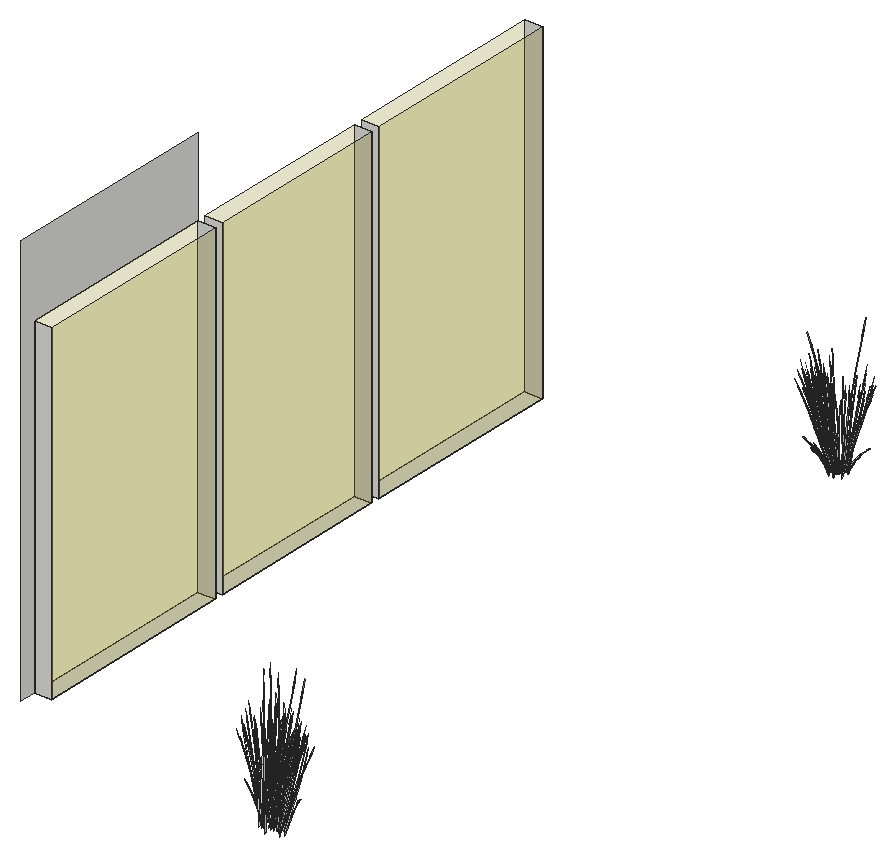
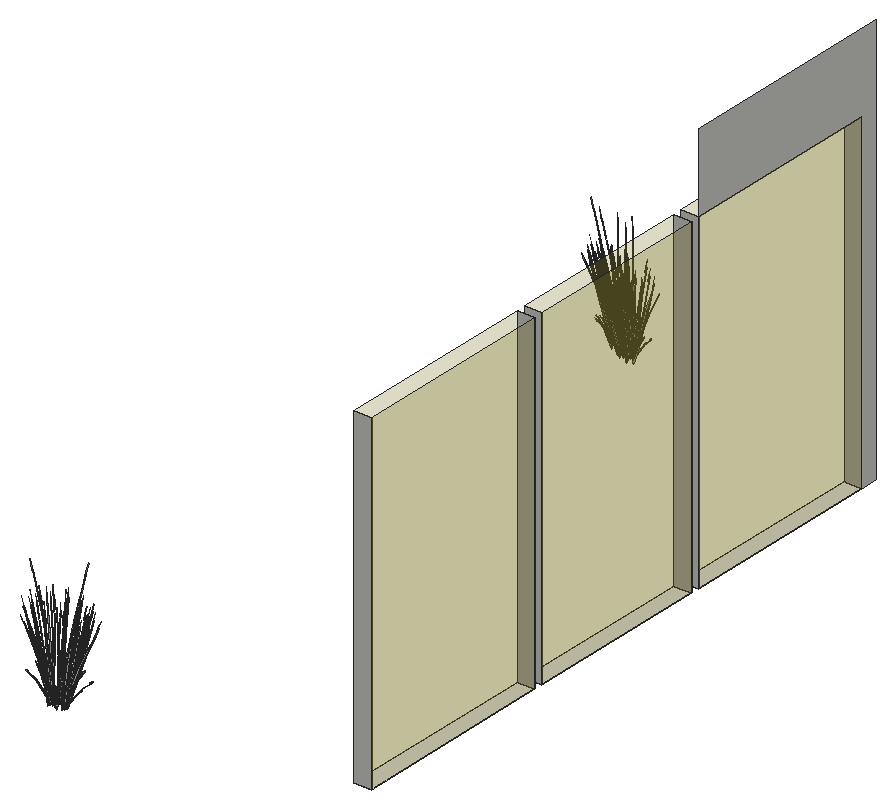
# SketchUp Ruby script. Lengths in inches.
U = 1.inch
M = Sketchup.active_model
def pt(a) = Geom::Point3d.new(a.map { |v| v * U })
def face(e, loops, mat)
  f = e.add_face(loops[0].map { |a| pt(a) })
  loops[1..].each { |l| e.add_face(l.map { |a| pt(a) }).erase! }
  f.material = f.back_material = mat if mat
  f
end
# faces: each face lists its corners as indices into pts; further lists are holes
def faces(e, pts, list, mat = nil) = list.each { |f| face(e, (f[0].is_a?(Array) ? f : [f]).map { |l| l.map { |i| pts[i] } }, mat) }
# xy, xz, yz: faces in a plane at the given z, y or x. An outline is a flat list of corners, or four numbers for a rectangle; further outlines are holes
def ring(l) = l.size == 4 ? [[l[0], l[1]], [l[2], l[1]], [l[2], l[3]], [l[0], l[3]]] : l.each_slice(2).to_a
def flat(e, list, mat, &to3) = list.each { |f| face(e, (f[0].is_a?(Array) ? f : [f]).map { |l| ring(l).map { |u, v| to3.(u, v) } }, mat) }
def xy(e, z, list, mat = nil) = flat(e, list, mat) { |x, y| [x, y, z] }
def xz(e, y, list, mat = nil) = flat(e, list, mat) { |x, z| [x, y, z] }
def yz(e, x, list, mat = nil) = flat(e, list, mat) { |y, z| [x, y, z] }
def lines(e, pts, list) = list.each { |a, b| e.add_line(pt(pts[a]), pt(pts[b])) }
# prism: a flat outline (further loops are holes) pulled along v
def prism(e, loops, v, mat = nil)
  f = face(e, loops, mat); d = Geom::Vector3d.new(v.map { |x| x * U })
  f.pushpull(f.normal.samedirection?(d) ? d.length : -d.length)
end
def box(e, o, s, mat = nil) = prism(e, [[o, [o[0] + s[0], o[1], o[2]], [o[0] + s[0], o[1] + s[1], o[2]], [o[0], o[1] + s[1], o[2]]]], [0, 0, s[2]], mat)
def at(x, y, z, deg = 0) = Geom::Transformation.translation(pt([x, y, z])) * Geom::Transformation.rotation(ORIGIN, Z_AXIS, deg.degrees)
def axes(o, x, y, z) = Geom::Transformation.new([*x, 0, *y, 0, *z, 0, *pt(o).to_a, 1])
def part(name) = M.definitions.add(name)
# library, detail: a bought-in or finely detailed component or shape, given as its bounding box
def library(name, o, s) = part(name).tap { |d| box(d.entities, o, s) }
def detail(e, o, s) = box(e.add_group.entities, o, s)
def put(e, d, t, mat = nil) = e.add_instance(d, t).tap { |i| i.material = mat if mat }
def group(e, t, mat = nil) = e.add_group.tap { |g| g.transformation = t; g.material = mat if mat }.entities
root = M.entities
M.materials.add("Glass_Basic_01").color = [186, 175, 42]
M.materials["Glass_Basic_01"].alpha = 0.25
M.materials.add("LightPink_Translucent").color = [144, 107, 117]
M.materials["LightPink_Translucent"].alpha = 0.75
c1 = part("blade")
p = [[2.15,0.21,22],[0,0.17,0],[0.09,0.45,0],[2.18,0.31,22],[2.29,0.31,22],[0.38,0.45,0],
  [2.48,0.24,33],[2.49,0.24,33],[2.48,0.22,33]]
faces(c1.entities,p,[[0,1,2,3],[4,5,2,3],[6,3,4,7],[8,0,3,6]])
c2 = part("seeds")
p = [[0.3,-0.1,1.38],[-0.01,-0.03,1.59],[-0.01,-0.03,0.03],[0.14,-0.07,-0.07],[0.29,-0.03,3],[0.15,0.01,3.11]]
faces(c2.entities,p,[[0,1,2,3],[1,0,4,5]],"LightPink_Translucent")
c3 = part("blade with seeds")
put(c3.entities,c1,at(0,0,0))
put(c3.entities,c2,axes([2.4,0.25,30.99],[1.5799,-0.05474,1.17369],[-0.12525,1.92788,0.29478],[-0.07173,-0.02425,1.56792]))
xy(root,51,[[241,49,247,119],[241,122,247,186],[241,189,247,259]])
xz(root,49,[[241,51,247,165]])
xz(root,119,[[241,51,247,165]])
xz(root,122,[[241,51,247,165]])
xz(root,186,[[241,51,247,165]])
xz(root,189,[[241,51,247,165]])
xz(root,259,[[241,51,247,165]])
yz(root,241,[[43,51,43,192,119,192,119,165,49,165,49,51]])
yz(root,241,[[49,51,119,165],[122,51,186,165],[189,51,259,165]],"Glass_Basic_01")
yz(root,247,[[49,51,119,165],[122,51,186,165],[189,51,259,165]],"Glass_Basic_01")
put(root,c3,axes([336.58,28.07,50.51],[-0.01379,-0.36791,1.24828],[0.62424,0.09537,0.52853],[-0.14764,0.20132,1.17828]))
put(root,c3,axes([336.63,29.49,52.14],[0.49824,-0.09289,-0.45151],[0.08716,0.35177,-0.34973],[0.13382,0.10081,0.86392]))
put(root,c3,axes([336.7,30.62,50.44],[0.21042,-0.1771,1.01491],[0.08303,0.28036,0.74569],[-0.15207,0.0502,0.22354]))
put(root,c3,axes([341.77,30.29,52],[0.28729,0.24465,-0.31292],[-0.32804,0.23159,0.40398],[0.16667,0.03524,0.77298]))
put(root,c3,axes([336.83,32.29,52.4],[0.44368,-0.17257,-0.62776],[0.24726,0.35524,0.07576],[0.21437,-0.04035,0.88802]))
put(root,c3,axes([337.49,29.85,52],[-0.43951,0.05584,-0.31292],[-0.11606,-0.31924,0.40398],[-0.12595,0.08575,0.77298]))
put(root,c3,axes([334,28.74,51.43],[0.09401,-0.13431,1.51428],[0.3944,0.27795,0.12244],[-0.17792,0.17323,0.64734]))
put(root,c3,axes([340.73,29.67,51.43],[-0.18755,-0.06732,1.51428],[0.38813,-0.28243,0.12244],[0.24191,0.12741,0.64734]))
put(root,c3,axes([340.77,28.78,51.95],[-0.4363,-0.20303,1.22187],[0.46069,-0.31611,0.5272],[0.14077,0.1905,1.18105]))
put(root,c3,axes([334.11,29.5,52],[-0.34164,0.20573,-0.31292],[-0.3234,-0.23491,0.40398],[-0.04921,0.11936,0.77298]))
put(root,c3,axes([335.1,29.67,52.45],[0.49409,-0.18193,-0.10745],[0.24281,0.32289,-0.59638],[0.06519,0.13607,0.90619]))
put(root,c3,axes([337.625,29.64,52.45],[0.46706,0.21546,-0.10745],[-0.26908,0.31203,-0.59638],[-0.13196,0.10846,0.90619]))
put(root,c3,axes([341.43,30.43,50.44],[-0.28429,-0.11236,1.01491],[0.36709,-0.11416,0.74569],[0.09901,0.0967,0.22354]))
put(root,c3,axes([334.33,30.3,50.44],[-0.01307,-0.23234,1.01491],[0.32652,0.16572,0.74569],[-0.06422,0.11074,0.22354]))
put(root,c3,axes([337.21,32.32,52],[0.41962,0.10901,-0.31292],[-0.12239,0.31802,0.40398],[0.16894,-0.02916,0.77298]))
put(root,c3,axes([340.43,30.75,52.45],[0.30087,-0.33447,-0.10745],[0.43572,0.19269,-0.59638],[0.15146,0.0945,0.90619]))
put(root,c3,axes([338.25,29.54,51.43],[0.12611,-0.12006,1.51428],[0.31843,0.32408,0.12244],[-0.2184,0.14759,0.64734]))
put(root,c3,axes([332.27,31.82,52],[-0.41962,-0.10901,-0.31292],[0.12239,-0.31802,0.40398],[-0.16894,0.02916,0.77298]))
put(root,c3,axes([337.86,29.89,52.14],[0.12971,0.3568,-0.45151],[-0.49122,0.06241,-0.34973],[-0.14077,0.09583,0.86392]))
put(root,c3,axes([334.45,29.4,52.42],[0.36145,0.26255,-0.50118],[-0.38183,0.22994,-0.3882],[-0.055,0.1334,0.95895]))
put(root,c3,axes([336.0625,31.93,51.43],[-0.20943,0.00885,1.51428],[0.13893,-0.38357,0.12244],[0.29846,0.02372,0.64734]))
put(root,c3,axes([340.74,29.17,50.51],[-0.01379,-0.36791,1.24828],[0.62424,0.09537,0.52853],[-0.14764,0.20132,1.17828]))
put(root,c3,axes([335.52,29.66,52.14],[0.49634,0.09796,-0.45151],[-0.17013,0.33585,-0.34973],[0.04551,0.13522,0.86392]))
put(root,c3,axes([335.8,28.96,51.43],[-0.11542,-0.12546,1.51428],[0.53333,-0.10562,0.12244],[0.12054,0.19696,0.64734]))
put(root,c3,axes([340.79,30.59,52.14],[0.49824,-0.09289,-0.45151],[0.08716,0.35177,-0.34973],[0.13382,0.10081,0.86392]))
put(root,c3,axes([335.3,29.86,52],[-0.15222,0.30049,-0.31292],[-0.44409,-0.08764,0.40398],[0.04072,0.12098,0.77298]))
put(root,c3,axes([334.34,29.28,52.72],[-0.01314,0.36145,-0.69681],[-0.55324,-0.02428,0.08409],[-0.05838,0.15313,0.9857]))
put(root,c3,axes([334.86,29.03,51.43],[-0.01236,-0.14998,1.51428],[0.53562,0.09949,0.12244],[-0.03313,0.21373,0.64734]))
put(root,c3,axes([333.55,31.76,50.95],[0.14352,-0.05653,1.56454],[0.04949,0.39467,0.12244],[-0.31087,0.05237,0.55918]))
put(root,c3,axes([338.1,32.39,50.44],[-0.31197,0.06451,1.01491],[0.14684,-0.26661,0.74569],[0.1655,0.01824,0.22354]))
put(root,c3,axes([338.16,29.84,51.43],[0.09401,-0.13431,1.51428],[0.3944,0.27795,0.12244],[-0.17792,0.17323,0.64734]))
put(root,c3,axes([335.34,29.59,52.4],[0.24099,0.31773,-0.62776],[-0.49607,0.17707,0.07576],[0.05635,0.15352,0.88802]))
put(root,c3,axes([338.27,30.59,52],[-0.34164,0.20573,-0.31292],[-0.3234,-0.23491,0.40398],[-0.04921,0.11936,0.77298]))
put(root,c3,axes([339.25,30.77,52.45],[0.49409,-0.18193,-0.10745],[0.24281,0.32289,-0.59638],[0.06519,0.13607,0.90619]))
put(root,c3,axes([332.01,32.03,52.17],[-0.08245,0.05073,1.54581],[0.00701,0.37067,-0.24447],[-0.18899,0.0482,0.12397]))
put(root,c3,axes([332.5625,31.98,52.14],[-0.13679,0.35544,-0.45151],[-0.46898,-0.12183,-0.34973],[-0.18882,0.03259,0.86392]))
put(root,c3,axes([332.54,31.67,52.45],[0.25405,0.35383,-0.10745],[-0.45089,0.17388,-0.59638],[-0.19001,0.04668,0.90619]))
put(root,c3,axes([337.55,33.21,51.47],[-0.09664,-0.32847,-0.03085],[0.45676,-0.07551,-0.13989],[0.09538,0.02082,0.4614]))
put(root,c3,axes([338.48,31.39,50.44],[-0.01307,-0.23234,1.01491],[0.32652,0.16572,0.74569],[-0.06422,0.11074,0.22354]))
put(root,c3,axes([336.37,33.2,52.45],[0.02704,-0.39739,-0.10745],[0.51189,0.01086,-0.59638],[0.19715,0.0276,0.90619]))
put(root,c3,axes([338.61,30.5,52.42],[0.36145,0.26255,-0.50118],[-0.38183,0.22994,-0.3882],[-0.055,0.1334,0.95895]))
put(root,c3,axes([339.68,30.75,52.14],[0.49634,0.09796,-0.45151],[-0.17013,0.33585,-0.34973],[0.04551,0.13522,0.86392]))
put(root,c3,axes([334.15,29.79,50.97],[0.01109,-0.20172,1.3638],[0.49896,0.10655,0.18846],[-0.04323,0.21498,0.64398]))
put(root,c3,axes([339.96,30.06,51.43],[-0.11542,-0.12546,1.51428],[0.53333,-0.10562,0.12244],[0.12054,0.19696,0.64734]))
put(root,c3,axes([339.45,30.96,52],[-0.15222,0.30049,-0.31292],[-0.44409,-0.08764,0.40398],[0.04072,0.12098,0.77298]))
put(root,c3,axes([336.82,32.96,52.17],[0.10831,-0.00661,1.54581],[0.29709,-0.30358,-0.24447],[0.19266,0.04007,0.12397]))
put(root,c3,axes([338.49,30.375,52.72],[-0.01314,0.36145,-0.69681],[-0.55324,-0.02428,0.08409],[-0.05838,0.15313,0.9857]))
put(root,c3,axes([332.55,32.16,51.43],[0.17519,-0.08265,1.51428],[0.14749,0.38193,0.12244],[-0.27504,0.08632,0.64734]))
put(root,c3,axes([339.02,30.12,51.43],[-0.01236,-0.14998,1.51428],[0.53562,0.09949,0.12244],[-0.03313,0.21373,0.64734]))
put(root,c3,axes([336.4,33.01,52.4],[0.50473,0.00941,-0.62776],[-0.0339,0.39618,0.07576],[0.21383,0.04181,0.88802]))
put(root,c3,axes([339.5,30.6875,52.4],[0.24099,0.31773,-0.62776],[-0.49607,0.17707,0.07576],[0.05635,0.15352,0.88802]))
put(root,c3,axes([331.63,33.5,50.44],[0.21042,-0.1771,1.01491],[0.08303,0.28036,0.74569],[-0.15207,0.0502,0.22354]))
put(root,c3,axes([336.7,33.17,52],[0.28729,0.24465,-0.31292],[-0.32804,0.23159,0.40398],[0.16667,0.03524,0.77298]))
put(root,c3,axes([332.43,32.73,52],[-0.43951,0.05584,-0.31292],[-0.11606,-0.31924,0.40398],[-0.12595,0.08575,0.77298]))
put(root,c3,axes([338.31,30.89,50.97],[0.01109,-0.20172,1.3638],[0.49896,0.10655,0.18846],[-0.04323,0.21498,0.64398]))
put(root,c3,axes([335.67,32.54,51.43],[-0.18755,-0.06732,1.51428],[0.38813,-0.28243,0.12244],[0.24191,0.12741,0.64734]))
put(root,c3,axes([335.7,31.66,51.95],[-0.4363,-0.20303,1.22187],[0.46069,-0.31611,0.5272],[0.14077,0.1905,1.18105]))
put(root,c3,axes([332.56,32.51,52.45],[0.46706,0.21546,-0.10745],[-0.26908,0.31203,-0.59638],[-0.13196,0.10846,0.90619]))
put(root,c3,axes([336.36,33.3125,50.44],[-0.28429,-0.11236,1.01491],[0.36709,-0.11416,0.74569],[0.09901,0.0967,0.22354]))
put(root,c3,axes([335.36,33.63,52.45],[0.30087,-0.33447,-0.10745],[0.43572,0.19269,-0.59638],[0.15146,0.0945,0.90619]))
put(root,c3,axes([333.1875,32.42,51.43],[0.12611,-0.12006,1.51428],[0.31843,0.32408,0.12244],[-0.2184,0.14759,0.64734]))
put(root,c3,axes([332.79,32.77,52.14],[0.12971,0.3568,-0.45151],[-0.49122,0.06241,-0.34973],[-0.14077,0.09583,0.86392]))
put(root,c3,axes([335.67,32.05,50.51],[-0.01379,-0.36791,1.24828],[0.62424,0.09537,0.52853],[-0.14764,0.20132,1.17828]))
put(root,c3,axes([335.72,33.47,52.14],[0.49824,-0.09289,-0.45151],[0.08716,0.35177,-0.34973],[0.13382,0.10081,0.86392]))
put(root,c3,axes([333.09,32.71,51.43],[0.09401,-0.13431,1.51428],[0.3944,0.27795,0.12244],[-0.17792,0.17323,0.64734]))
put(root,c3,axes([333.2,33.47,52],[-0.34164,0.20573,-0.31292],[-0.3234,-0.23491,0.40398],[-0.04921,0.11936,0.77298]))
put(root,c3,axes([332.02,33.41,52.17],[-0.01255,0.07733,1.54581],[0.35618,0.269,-0.24447],[-0.09325,0.12721,0.12397]))
put(root,c3,axes([334.1875,33.65,52.45],[0.49409,-0.18193,-0.10745],[0.24281,0.32289,-0.59638],[0.06519,0.13607,0.90619]))
put(root,c3,axes([333.42,34.27,50.44],[-0.01307,-0.23234,1.01491],[0.32652,0.16572,0.74569],[-0.06422,0.11074,0.22354]))
put(root,c3,axes([333.54,33.375,52.42],[0.36145,0.26255,-0.50118],[-0.38183,0.22994,-0.3882],[-0.055,0.1334,0.95895]))
put(root,c3,axes([334.61,33.63,52.14],[0.49634,0.09796,-0.45151],[-0.17013,0.33585,-0.34973],[0.04551,0.13522,0.86392]))
put(root,c3,axes([334.89,32.9375,51.43],[-0.11542,-0.12546,1.51428],[0.53333,-0.10562,0.12244],[0.12054,0.19696,0.64734]))
put(root,c3,axes([334.39,33.84,52],[-0.15222,0.30049,-0.31292],[-0.44409,-0.08764,0.40398],[0.04072,0.12098,0.77298]))
put(root,c3,axes([333.43,33.25,52.72],[-0.01314,0.36145,-0.69681],[-0.55324,-0.02428,0.08409],[-0.05838,0.15313,0.9857]))
put(root,c3,axes([333.95,33,51.43],[-0.01236,-0.14998,1.51428],[0.53562,0.09949,0.12244],[-0.03313,0.21373,0.64734]))
put(root,c3,axes([334.43,33.57,52.4],[0.24099,0.31773,-0.62776],[-0.49607,0.17707,0.07576],[0.05635,0.15352,0.88802]))
put(root,c3,axes([334.07,34.37,52.17],[0.064,0.06292,1.54581],[0.51651,0.02472,-0.24447],[0.05194,0.13877,0.12397]))
put(root,c3,axes([333.24,33.76,50.97],[0.01109,-0.20172,1.3638],[0.49896,0.10655,0.18846],[-0.04323,0.21498,0.64398]))
put(root,c3,axes([332.69,275.14,51.43],[0.11542,0.12546,1.51428],[-0.53333,0.10562,0.12244],[-0.12054,-0.19696,0.64734]))
put(root,c3,axes([333.57,274.3,52.17],[-0.07723,-0.05479,1.54581],[-0.51538,0.03473,-0.24447],[-0.08225,-0.13104,0.12397]))
put(root,c3,axes([334.11,275.23,52.4],[-0.24099,-0.31773,-0.62776],[0.49607,-0.17707,0.07576],[-0.05635,-0.15352,0.88802]))
put(root,c3,axes([335.12,275.54,52.4],[0.01314,-0.36145,-0.62776],[0.55324,0.02428,0.07576],[0.05838,-0.15313,0.88802]))
put(root,c3,axes([335.89,274.98,52.17],[-0.00487,-0.07777,1.54581],[-0.41166,-0.22476,-0.24447],[0.06364,-0.13625,0.12397]))
put(root,c3,axes([334.16,274.96,52],[0.15222,-0.30049,-0.31292],[0.44409,0.08764,0.40398],[-0.04072,-0.12098,0.77298]))
put(root,c3,axes([334.5,275.36,51.43],[-0.09401,0.13431,1.51428],[-0.3944,-0.27795,0.12244],[0.17792,-0.17323,0.64734]))
put(root,c3,axes([333.93,275.17,52.14],[-0.49634,-0.09796,-0.45151],[0.17013,-0.33585,-0.34973],[-0.04551,-0.13522,0.86392]))
put(root,c3,axes([334.24,274.33,50.44],[0.06477,0.22786,1.01491],[-0.35932,-0.1262,0.74569],[0.03867,-0.11667,0.22354]))
put(root,c3,axes([335.01,275.42,52.14],[-0.36145,-0.26255,-0.45151],[0.38183,-0.22994,-0.34973],[0.055,-0.1334,0.86392]))
put(root,c3,axes([334.36,275.15,52.45],[-0.49409,0.18193,-0.10745],[-0.24281,-0.32289,-0.59638],[-0.06519,-0.13607,0.90619]))
put(root,c3,axes([335.38,275.56,52.45],[-0.55492,-0.01936,-0.10745],[0.01517,-0.36657,-0.59638],[0.03855,-0.14118,0.90619]))
put(root,c3,axes([335.35,275.32,52],[0.34164,-0.20573,-0.31292],[0.3234,0.23491,0.40398],[0.04921,-0.11936,0.77298]))
put(root,c3,axes([332.39,274.6,50.44],[0.26338,0.136,1.01491],[-0.38358,0.08175,0.74569],[-0.08207,-0.10452,0.22354]))
put(root,c3,axes([333.03,275.32,52.4],[-0.43054,-0.18887,-0.62776],[0.30598,-0.33097,0.07576],[-0.15599,-0.11277,0.88802]))
put(root,c3,axes([332.88,275.07,52],[-0.07798,-0.31474,-0.31292],[0.44579,-0.08311,0.40398],[-0.11974,-0.09019,0.77298]))
put(root,c3,axes([331.92,275.53,51.43],[0.18755,0.06732,1.51428],[-0.38813,0.28243,0.12244],[-0.24191,-0.12741,0.64734]))
put(root,c3,axes([332.83,275.33,52.14],[-0.49824,0.09289,-0.45151],[-0.08716,-0.35177,-0.34973],[-0.13382,-0.10081,0.86392]))
put(root,c3,axes([335.77,276.17,52.4],[0.26374,-0.30832,-0.62776],[0.46217,0.21911,0.07576],[0.15748,-0.11171,0.88802]))
put(root,c3,axes([335.76,276.03,52.14],[-0.12971,-0.3568,-0.45151],[0.49122,-0.06241,-0.34973],[0.14077,-0.09583,0.86392]))
put(root,c3,axes([331.88,274.91,52.17],[-0.10864,-0.00276,1.54581],[-0.34587,0.27582,-0.24447],[-0.18454,-0.05636,0.12397]))
put(root,c3,axes([335.99,276.28,52.45],[-0.46706,-0.21546,-0.10745],[0.26908,-0.31203,-0.59638],[0.13196,-0.10846,0.90619]))
put(root,c3,axes([334.06,277.46,50.9375],[0.43633,0.15757,1.33654],[-0.42745,0.33945,0.52853],[-0.19146,-0.20119,1.12046]))
put(root,c3,axes([336.36,275.32,50.44],[-0.16818,0.19891,1.01491],[-0.14456,-0.26725,0.74569],[0.1389,-0.06697,0.22354]))
put(root,c3,axes([336.12,276.0625,52],[0.43951,-0.05584,-0.31292],[0.11606,0.31924,0.40398],[0.12595,-0.08575,0.77298]))
put(root,c3,axes([331.85,275.625,52],[-0.28729,-0.24465,-0.31292],[0.32804,-0.23159,0.40398],[-0.16667,-0.03524,0.77298]))
put(root,c3,axes([332.15,275.79,52.4],[-0.50473,-0.00941,-0.62776],[0.0339,-0.39618,0.07576],[-0.21383,-0.04181,0.88802]))
put(root,c3,axes([337.39,276.57,52.17],[0.07006,-0.05952,1.54581],[-0.08968,-0.3651,-0.24447],[0.1758,-0.06922,0.12397]))
put(root,c3,axes([331.98,275.87,52.14],[-0.36663,0.25884,-0.45151],[-0.32109,-0.27343,-0.34973],[-0.18628,-0.03938,0.86392]))
put(root,c3,axes([332.18,275.6,52.45],[-0.02704,0.39739,-0.10745],[-0.51189,-0.01086,-0.59638],[-0.19715,-0.0276,0.90619]))
put(root,c3,axes([336.01,277.12,52.45],[-0.25405,-0.35383,-0.10745],[0.45089,-0.17388,-0.59638],[0.19001,-0.04668,0.90619]))
put(root,c3,axes([335.98,276.82,52.14],[0.13679,-0.35544,-0.45151],[0.46898,0.12183,-0.34973],[0.18882,-0.03259,0.86392]))
put(root,c3,axes([331.52,276.14,51.43],[0.20943,-0.00885,1.51428],[-0.13893,0.38357,0.12244],[-0.29846,-0.02372,0.64734]))
put(root,c3,axes([335.9,276.95,52.4],[0.44368,-0.17257,-0.62776],[0.24726,0.35524,0.07576],[0.21437,-0.04035,0.88802]))
put(root,c3,axes([336.27,276.98,52],[0.41962,0.10901,-0.31292],[-0.12239,0.31802,0.40398],[0.16894,-0.02916,0.77298]))
put(root,c3,axes([331.34,276.47,52],[-0.41962,-0.10901,-0.31292],[0.12239,-0.31802,0.40398],[-0.16894,0.02916,0.77298]))
put(root,c3,axes([335.13,276.59,51.43],[-0.20943,0.00885,1.51428],[0.13893,-0.38357,0.12244],[0.29846,0.02372,0.64734]))
put(root,c3,axes([332.62,276.42,50.95],[0.14352,-0.05653,1.56454],[0.04949,0.39467,0.12244],[-0.31087,0.05237,0.55918]))
put(root,c3,axes([331.08,276.68,52.17],[-0.08245,0.05073,1.54581],[0.00701,0.37067,-0.24447],[-0.18899,0.0482,0.12397]))
put(root,c3,axes([331.63,276.64,52.14],[-0.13679,0.35544,-0.45151],[-0.46898,-0.12183,-0.34973],[-0.18882,0.03259,0.86392]))
put(root,c3,axes([331.61,276.33,52.45],[0.25405,0.35383,-0.10745],[-0.45089,0.17388,-0.59638],[-0.19001,0.04668,0.90619]))
put(root,c3,axes([336.62,277.87,51.47],[-0.09664,-0.32847,-0.03085],[0.45676,-0.07551,-0.13989],[0.09538,0.02082,0.4614]))
put(root,c3,axes([335.4375,277.86,52.45],[0.02704,-0.39739,-0.10745],[0.51189,0.01086,-0.59638],[0.19715,0.0276,0.90619]))
put(root,c3,axes([335.88,277.62,52.17],[0.10831,-0.00661,1.54581],[0.29709,-0.30358,-0.24447],[0.19266,0.04007,0.12397]))
put(root,c3,axes([331.61,276.82,51.43],[0.17519,-0.08265,1.51428],[0.14749,0.38193,0.12244],[-0.27504,0.08632,0.64734]))
put(root,c3,axes([335.46,277.67,52.4],[0.50473,0.00941,-0.62776],[-0.0339,0.39618,0.07576],[0.21383,0.04181,0.88802]))
put(root,c3,axes([335.77,277.83,52],[0.28729,0.24465,-0.31292],[-0.32804,0.23159,0.40398],[0.16667,0.03524,0.77298]))
put(root,c3,axes([331.49,277.39,52],[-0.43951,0.05584,-0.31292],[-0.11606,-0.31924,0.40398],[-0.12595,0.08575,0.77298]))
put(root,c3,axes([334.73,277.2,51.43],[-0.18755,-0.06732,1.51428],[0.38813,-0.28243,0.12244],[0.24191,0.12741,0.64734]))
put(root,c3,axes([334.77,276.32,51.95],[-0.4363,-0.20303,1.22187],[0.46069,-0.31611,0.5272],[0.14077,0.1905,1.18105]))
put(root,c3,axes([331.625,277.17,52.45],[0.46706,0.21546,-0.10745],[-0.26908,0.31203,-0.59638],[-0.13196,0.10846,0.90619]))
put(root,c3,axes([334.43,278.29,52.45],[0.30087,-0.33447,-0.10745],[0.43572,0.19269,-0.59638],[0.15146,0.0945,0.90619]))
put(root,c3,axes([332.25,277.08,51.43],[0.12611,-0.12006,1.51428],[0.31843,0.32408,0.12244],[-0.2184,0.14759,0.64734]))
put(root,c3,axes([331.86,277.43,52.14],[0.12971,0.3568,-0.45151],[-0.49122,0.06241,-0.34973],[-0.14077,0.09583,0.86392]))
